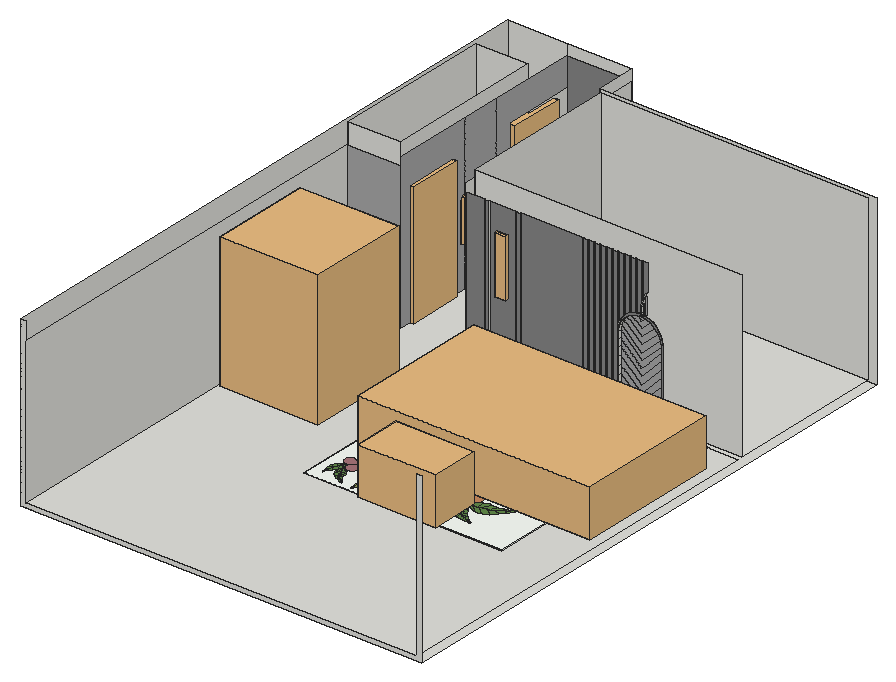
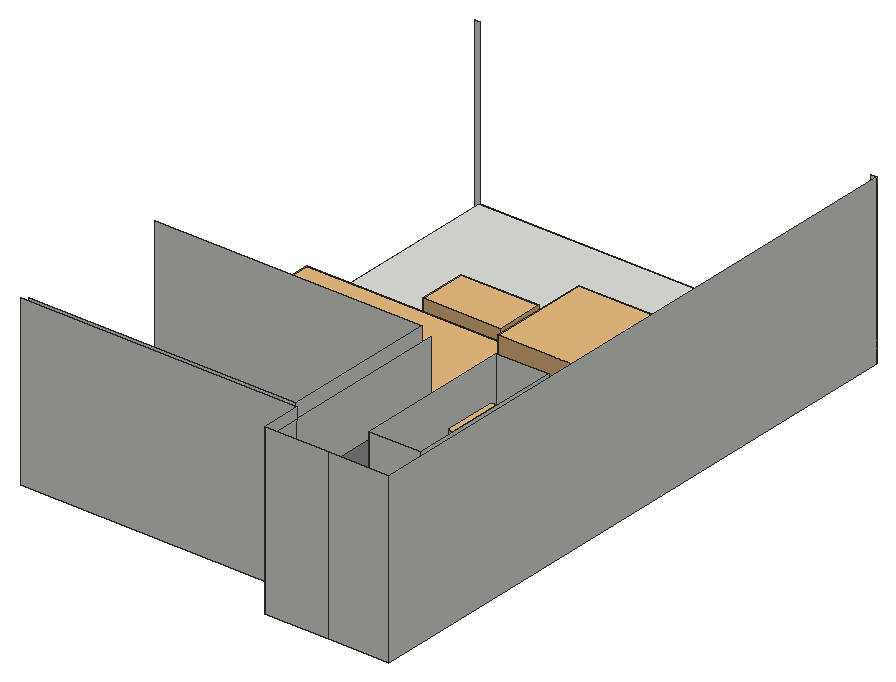
# SketchUp Ruby script. Lengths in inches.
U = 1.inch
M = Sketchup.active_model
def pt(a) = Geom::Point3d.new(a.map { |v| v * U })
def face(e, loops, mat)
  f = e.add_face(loops[0].map { |a| pt(a) })
  loops[1..].each { |l| e.add_face(l.map { |a| pt(a) }).erase! }
  f.material = f.back_material = mat if mat
  f
end
# faces: each face lists its corners as indices into pts; further lists are holes
def faces(e, pts, list, mat = nil) = list.each { |f| face(e, (f[0].is_a?(Array) ? f : [f]).map { |l| l.map { |i| pts[i] } }, mat) }
# xy, xz, yz: faces in a plane at the given z, y or x. An outline is a flat list of corners, or four numbers for a rectangle; further outlines are holes
def ring(l) = l.size == 4 ? [[l[0], l[1]], [l[2], l[1]], [l[2], l[3]], [l[0], l[3]]] : l.each_slice(2).to_a
def flat(e, list, mat, &to3) = list.each { |f| face(e, (f[0].is_a?(Array) ? f : [f]).map { |l| ring(l).map { |u, v| to3.(u, v) } }, mat) }
def xy(e, z, list, mat = nil) = flat(e, list, mat) { |x, y| [x, y, z] }
def xz(e, y, list, mat = nil) = flat(e, list, mat) { |x, z| [x, y, z] }
def yz(e, x, list, mat = nil) = flat(e, list, mat) { |y, z| [x, y, z] }
def lines(e, pts, list) = list.each { |a, b| e.add_line(pt(pts[a]), pt(pts[b])) }
# prism: a flat outline (further loops are holes) pulled along v
def prism(e, loops, v, mat = nil)
  f = face(e, loops, mat); d = Geom::Vector3d.new(v.map { |x| x * U })
  f.pushpull(f.normal.samedirection?(d) ? d.length : -d.length)
end
def box(e, o, s, mat = nil) = prism(e, [[o, [o[0] + s[0], o[1], o[2]], [o[0] + s[0], o[1] + s[1], o[2]], [o[0], o[1] + s[1], o[2]]]], [0, 0, s[2]], mat)
def at(x, y, z, deg = 0) = Geom::Transformation.translation(pt([x, y, z])) * Geom::Transformation.rotation(ORIGIN, Z_AXIS, deg.degrees)
def axes(o, x, y, z) = Geom::Transformation.new([*x, 0, *y, 0, *z, 0, *pt(o).to_a, 1])
def part(name) = M.definitions.add(name)
# library, detail: a bought-in or finely detailed component or shape, given as its bounding box
def library(name, o, s) = part(name).tap { |d| box(d.entities, o, s) }
def detail(e, o, s) = box(e.add_group.entities, o, s)
def put(e, d, t, mat = nil) = e.add_instance(d, t).tap { |i| i.material = mat if mat }
def group(e, t, mat = nil) = e.add_group.tap { |g| g.transformation = t; g.material = mat if mat }.entities
root = M.entities
M.materials.add("[0013_LightCoral]").color = [251, 255, 248]
M.materials.add("[0013_LightCoral]1").color = [240, 128, 128]
M.materials.add("[0132_LightGray]").color = [135, 135, 135]
M.materials.add("[0132_LightGray]1").color = [169, 169, 169]
M.materials.add("[Fabric Linen]").color = [168, 116, 117]
M.materials.add("[Granite Tile]").color = [201, 139, 95]
M.materials.add("[Vegetation Blur 01]").color = [168, 117, 122]
M.materials.add("[Vegetation Grass Artificial]").color = [98, 140, 74]
M.materials.add("[Vegetation Grass]").color = [144, 160, 91]
c1 = library("Dining+table+4+seater",[21.1,70.47,0],[72.14,73.92,98.58])
c2 = library("door (1)",[38.93,25.48,0],[40,9.94,82.68])
c3 = library("Succulent+decoration+(1)",[22.63,43.09,0],[32.53,2.35,30.92])
c4 = part("Group\#33")
xy(c4.entities,0,[[3.16,0,2.86,0.82,1.26,2.77,0,5.57,0.11,6.86,0.4375,6.76,0.52,6.68,0.63,6.49,1.02,6.09,1.86,5.44,2.36,5.07,2.77,4.84,3.39,4.72,3.7,4.65,4.07,4.27,3.85,2.85,3.75,2.45],[3.16,0,3.75,2.45,4.12,2.5,4.33,2.64,4.83,2.9,6,3.45,6.93,3.96,7.42,4.13,7.62,4.24,7.93,4.17,7.65,3.64,5.62,1.44],[3.75,2.45,3.85,2.85,4.07,4.27,4.28,5.69,4.62,5.72,4.99,5.91,5.7,6.28,6.96,7,8.1,7.62,9.16,8.86,9.08,6.35,8.01,4.32,7.93,4.17,7.62,4.24,7.42,4.13,6.93,3.96,6,3.45,4.83,2.9,4.33,2.64,4.12,2.5],[4.07,4.27,3.7,4.65,3.39,4.72,2.77,4.84,2.36,5.07,1.86,5.44,1.02,6.09,0.63,6.49,0.52,6.68,0.4375,6.76,0.11,6.86,0.14,7.22,0.28,8.87,0.86,10.33,1.05,9.89,1.35,9.64,1.86,9.3125,2.43,9.02,2.94,8.61,3.51,7.66,3.92,7.21,4.43,6.89,4.28,5.69],[4.28,5.69,4.43,6.89,4.58,8.08,4.59,8.84,4.91,8.96,5.15,9.24,5.74,9.79,6.26,10.125,6.8,10.3125,7.37,10.58,7.8,10.9,8.23,11.24,8.64,11.89,9.16,8.86,8.1,7.62,6.96,7,5.7,6.28,4.99,5.91,4.62,5.72],
  [4.43,6.89,3.92,7.21,3.51,7.66,2.94,8.61,2.43,9.02,1.86,9.3125,1.35,9.64,1.05,9.89,0.86,10.33,1.44,11.8,1.87,13.11,2.28,13.24,2.5,13.125,2.83,12.88,3.0625,12.74,3.16,12.51,3.3,12.2,3.96,11.625,4.28,11.32,4.5,11.15,4.6,11.16,4.61,10.45,4.59,8.84,4.58,8.08],[4.59,8.84,4.61,10.45,4.6,11.16,4.58,12.86,4.66,13.19,4.88,13.24,5.22,13.32,5.85,13.71,6.06,14.02,6.21,14.38,6.39,14.7,6.78,15.17,7.14,14.6,8.64,11.89,8.23,11.24,7.8,10.9,7.37,10.58,6.8,10.3125,6.26,10.125,5.74,9.79,5.15,9.24,4.91,8.96],[4.5,11.15,4.28,11.32,3.96,11.625,3.3,12.2,3.16,12.51,3.0625,12.74,2.83,12.88,2.5,13.125,2.28,13.24,1.87,13.11,2.29,14.41,2.4,16.15,3.04,16.01,3.53,15.76,4.54,15.27,4.58,12.86,4.6,11.16],[4.58,12.86,4.54,15.27,3.82,17.41,3.98,17.35,4.0625,17.43,4.29,17.71,4.85,18.28,6.78,15.17,6.39,14.7,6.21,14.38,6.06,14.02,5.85,13.71,5.22,13.32,4.88,13.24,4.66,13.19],[4.54,15.27,3.53,15.76,3.04,16.01,2.4,16.15,2.51,17.89,2.36,19.5,3.27,19.22,3.62,18.5625,3.82,17.41],
  [3.98,17.35,3.82,17.41,3.62,18.5625,3.27,19.22,2.97,19.94,2.74,20.53,2.73,21.38,3.15,20.92,4.15,19.41,4.85,18.28,4.29,17.71,4.0625,17.43],[3.27,19.22,2.36,19.5,2.21,21.11,2.74,20.53,2.97,19.94],[2.74,20.53,2.21,21.11,2.22,21.31,2.1875,21.5,2.16,21.66,2.15,21.73,2.13,21.81,2.18,21.79,2.45,21.6,2.6,21.53,2.73,21.38]])
c5 = part("Group\#60")
g1 = group(c5.entities,at(9.35,11.87,0))
xy(g1,0,[[2.08,-11.87,1.91,-11.81,1.82,-11.79,1.73,-11.73,1.59,-11.28,1.96,-11.51,1.99,-11.61,2.03,-11.71,2.1,-11.85,2.1,-11.87],[1.73,-11.73,1.4375,-11.55,0.68,-10.9,0.14,-10.4,0.36,-10.02,0.43,-9.83,0.47,-9.78,0.56,-9.79,0.84,-10.37,1.12,-10.67,1.38,-11,1.59,-11.28],[1.96,-11.51,1.59,-11.28,1.38,-11,1.12,-10.67,1.64,-10.68],[1.64,-10.68,1.12,-10.67,0.84,-10.37,0.56,-9.79,-0.14,-8.76,0.47,-8.87,0.76,-8.93,1.125,-8.91,1.32,-9.85],[0.14,-10.4,-1.34,-9.04,-1.2,-8.73,-1.16,-8.54,-1.13,-8.32,-1.0625,-8.13,-0.79,-7.83,-0.62,-7.74,-0.51,-7.68,-0.52,-7.49,-0.14,-8.76,0.56,-9.79,0.47,-9.78,0.43,-9.83,0.36,-10.02],
  [-1.34,-9.04,-1.62,-8.79,-2.81,-7.58,-2.69,-7.17,-2.52,-6.93,-2.33,-6.69,-2.07,-6.47,-1.81,-6.29,-1.59,-6.04,-1.36,-5.66,-1.27,-5.47,-1.12,-5.36,-0.89,-6.22,-0.78,-6.59,-0.52,-7.49,-0.51,-7.68,-0.62,-7.74,-0.79,-7.83,-1.0625,-8.13,-1.13,-8.32,-1.16,-8.54,-1.2,-8.73],[0.76,-8.93,0.47,-8.87,-0.14,-8.76,-0.52,-7.49,-0.78,-6.59,-0.73,-6.57,-0.59,-6.63,-0.37,-6.74,0.0625,-6.95,0.18,-7.09,0.27,-7.2,0.41,-7.24,0.62,-7.32,0.75,-7.35,0.96,-7.22,0.92,-7.97,1.125,-8.91],[-2.81,-7.58,-3.54,-6.05,-3.16,-5.24,-2.65,-4.74,-2.09,-4.17,-1.77,-3.87,-1.6,-3.71,-1.42,-3.65,-1.33,-4.31,-1.23,-4.96,-1.12,-5.36,-1.27,-5.47,-1.36,-5.66,-1.59,-6.04,-1.81,-6.29,-2.07,-6.47,-2.33,-6.69,-2.52,-6.93,-2.69,-7.17],[0.75,-7.35,0.62,-7.32,0.41,-7.24,0.27,-7.2,0.18,-7.09,0.0625,-6.95,-0.37,-6.74,-0.59,-6.63,-0.73,-6.57,-0.78,-6.59,-0.89,-6.22,-1.12,-5.36,-1.23,-4.96,-1.33,-4.31,-1.01,-4.4,-0.72,-4.58,-0.28,-5,0.05,-5.14,0.4,-5.21,0.71,-5.31,0.91,-5.4,1.08,-5.6,0.99,-6.46,0.96,-7.22],[-3.54,-6.05,-3.87,-4.71,-3.6,-3.47,-3.58,-3.39,-3.41,-3.375,-3.32,-3.29,-3.08,-3.13,-2.67,-2.72,-2.13,-2.25,-1.9,-2.04,-1.8125,-1.9375,-1.625,-1.85,-1.62,-2.08,-1.52,-2.86,-1.42,-3.65,-1.6,-3.71,-1.77,-3.87,-2.09,-4.17,-2.65,-4.74,-3.16,-5.24],
  [1.08,-5.6,0.91,-5.4,0.71,-5.31,0.4,-5.21,0.05,-5.14,-0.28,-5,-0.72,-4.58,-1.01,-4.4,-1.33,-4.31,-1.42,-3.65,-1.52,-2.86,-1.27,-3.01,-1.09,-3,-0.75,-2.98,-0.5,-3.04,-0.18,-3.16,0.36,-3.375,0.63,-3.53,0.72,-3.61,0.77,-3.64,0.96,-3.65,1,-3.84,1.17,-4.74],[0.96,-3.65,0.77,-3.64,0.72,-3.61,0.63,-3.53,0.36,-3.375,-0.18,-3.16,-0.5,-3.04,-0.75,-2.98,-1.09,-3,-1.27,-3.01,-1.52,-2.86,-1.62,-2.08,-1.625,-1.85,-1.67,-0.47,-1.39,-0.86,-0.26,-1.66,0.83,-2.95],[-3.58,-3.39,-3.51,-3.0625,-2.76,-1.6,-1.67,-0.47,-1.625,-1.85,-1.8125,-1.9375,-1.9,-2.04,-2.13,-2.25,-2.67,-2.72,-3.08,-3.13,-3.32,-3.29,-3.41,-3.375]])
put(c5.entities,c4,axes([8.26,10.79,0],[-0.18907,0.36013,0],[-0.36013,-0.18907,0],[0,0,1]))
c6 = library("Group\#329",[0,0,0],[7.875,1.97,42.125])
c7 = part("Group\#34")
xy(c7.entities,0,[[9.92,0,2.48,3.46,1.45,4.25,0.66,5.28,0.17,6.47,0,7.76,0.17,9.04,0.66,10.24,1.45,11.26,2.48,12.05,3.68,12.55,4.96,12.72,6.24,12.55,7.44,12.05,8.47,11.26,9.26,10.24,9.75,9.04,9.92,7.76]])
c8 = part("Group\#36")
xy(c8.entities,0,[[9.92,0,2.48,3.46,1.45,4.25,0.66,5.28,0.17,6.47,0,7.76,0.17,9.04,0.66,10.24,1.45,11.26,2.48,12.05,3.68,12.55,4.96,12.72,6.24,12.55,7.44,12.05,8.47,11.26,9.26,10.24,9.75,9.04,9.92,7.76]])
c9 = part("Group\#38")
put(c9.entities,c4,at(-0.96,4.16,0,-54.9))
put(c9.entities,c4,at(0.46,7.11,0,4.699))
c10 = library("Throw pillow",[0,0,0],[9.42,19.46,15.55])
c11 = library("Group\#76",[0,0,0],[62.16,38.23,37.78])
c12 = library("sofa",[-89.99,-57.625,20.49],[181.58,106.54,46.48])
box(root,[107.14,126.82,3.125],[145.28,96.85,0.4375],"[0013_LightCoral]")
xy(root,0,[[0,0,44.125,447.875],[44.125,0,91.5625,447.875],[91.5625,0,295.1875,417.6875]])
xy(root,3.125,[[3.79,0,291.63,0,291.63,294.91,278.7,294.91,278.7,294.47,277.02,294.47,277.02,294.91,276.67,294.91,276.67,294.47,274.98,294.47,274.98,294.91,274.63,294.91,274.63,294.47,272.94,294.47,272.94,294.91,272.59,294.91,272.59,294.47,270.9,294.47,270.9,294.91,270.55,294.91,270.55,294.47,268.86,294.47,268.86,294.91,268.52,294.91,268.52,294.47,266.83,294.47,266.83,294.91,266.48,294.91,266.48,294.47,264.79,294.47,264.79,294.91,264.44,294.91,264.44,294.47,260.79,294.47,260.79,294.91,260.26,294.91,260.26,294.47,257.75,294.47,257.75,293.53,204.25,293.53,204.25,294.91,203.53,294.91,203.53,294.47,199.88,294.47,199.88,294.91,199.15,294.91,199.15,294.47,195.5,294.47,195.5,294.91,194.78,294.91,194.78,294.47,191.13,294.47,191.13,294.91,190.4,294.91,190.4,294.47,186.75,294.47,186.75,294.91,186.03,294.91,186.03,294.47,182.38,294.47,182.38,294.91,181.65,294.91,181.65,294.47,178,294.47,178,294.91,132.13,294.91,132.13,294.47,129.06,294.47,129.06,294.91,109.17,294.91,109.17,294.47,105.89,294.47,105.89,294.91,91.5625,294.91,91.5625,447.375,44.125,447.375,44.125,294.91,3.79,294.91],[2.9,297.81,41.22,414.79],[95.12,298.46,291.63,414.13],[41.22,302.6,44.125,342.1],[41.22,394.68,44.125,412.06]])
xy(root,4.38,[[205.51,293.53,236.48,294.91]],"[0132_LightGray]")
xy(root,74.29,[[216.65,293.53,216.66,294.91]])
xy(root,74.86,[[220.99,293.53,221.03,294.91]])
xz(root,0,[[0,0,295.1875,0,295.1875,123.125,291.63,123.125,291.63,3.125,3.79,3.125,3.79,123.125,0,123.125]])
xz(root,293.53,[[[204.25,3.125,237.73,3.125,237.73,58.125,237.16,62.46,236.33,64.45,235.49,66.49,233.34,69.3,232.83,69.96,230.15,72.02,229.36,72.62,227.05,73.58,225.4,74.26,225.32,74.29,225.04,74.33,222.99,74.6,222.32,74.6875,221.75,74.76,221.03,74.86,220.99,74.86,217.38,74.39,216.66,74.29,216.65,74.29,213,72.78,212.625,72.62,212.28,72.36,209.16,69.96,208.63,69.27,207.9,68.33,206.5,66.49,204.82,62.46,204.25,58.125],[205.51,4.38,205.51,58.04,206.04,62.13,207.59,65.86,208.9,67.5625,209.625,68.51,210.05,69.07,213.04,71.36,213.25,71.53,213.48,71.62,216.99,73.07,217.54,73.15,220.99,73.6,221.59,73.52,225,73.07,228.73,71.53,231.93,69.07,234.39,65.86,235.94,62.13,236.48,58.04,236.48,4.38]]],"[0132_LightGray]")
xz(root,294.47,[[105.89,3.125,109.17,109.39],[129.06,3.125,132.13,109.39],[178,3.125,181.65,109.39],[182.38,3.125,186.03,109.39],[186.75,3.125,190.4,109.39],
  [191.13,3.125,194.78,109.39],[195.5,3.125,199.15,109.39],[199.88,3.125,203.53,109.39],[204.25,58.125,204.82,62.46,206.5,66.49,207.9,68.33,207.9,109.39,204.25,109.39],[208.63,69.27,209.16,69.96,212.28,72.36,212.28,109.39,208.63,109.39],
  [213,72.78,216.65,74.29,216.65,109.39,213,109.39],[217.38,74.39,220.99,74.86,220.99,80.18,221.03,80.29,221.03,109.39,217.38,109.39],[221.75,82.74,222.51,85.27,225.4,89.72,225.4,109.39,221.75,109.39]],"[0132_LightGray]")
xz(root,294.66,[[225.04,74.33,225.04,86.79,223.69,84.72,223.11,82.79,223.11,74.58],[222.99,74.6,222.99,82.375,222.32,80.11,222.32,74.6875]],"[0132_LightGray]1")
xz(root,294.91,[[223.11,74.58,223.11,82.79,222.99,82.375,222.99,74.6],[220.99,74.86,221.03,74.86,221.03,80.29,220.99,80.18]])
xz(root,294.91,[[91.5625,3.125,105.89,109.39],[109.17,3.125,129.06,109.39],[132.13,3.125,178,109.39],[181.65,3.125,182.38,109.39],[186.03,3.125,186.75,109.39],
  [190.4,3.125,191.13,109.39],[194.78,3.125,195.5,109.39],[199.15,3.125,199.88,109.39],[203.53,3.125,204.25,109.39],[205.51,4.38,220.99,4.38,205.51,17.84],
  [220.99,4.38,236.48,17.84,236.48,25.84,220.99,10.29,205.51,23.88,205.51,17.84],[207.9,68.33,208.63,69.27,208.63,109.39,207.9,109.39],[212.28,72.36,212.625,72.62,213,72.78,213,109.39,212.28,109.39],[216.65,74.29,216.66,74.29,217.38,74.39,217.38,109.39,216.65,109.39],[221.03,80.29,221.75,82.74,221.75,109.39,221.03,109.39]],"[0132_LightGray]")
xz(root,294.91,[[3.79,3.125,44.125,109.39],[220.99,10.29,236.48,25.84,236.48,31.64,220.99,16.21,205.51,29.28,205.51,23.88],[220.99,16.21,236.48,31.64,236.48,37.31,220.99,21.66,205.51,35.56,205.51,29.28],[220.99,21.66,236.48,37.31,236.48,43.35,220.99,27.22,205.51,42.09,205.51,35.56],[220.99,27.22,236.48,43.35,236.48,48.5,220.99,32.74,205.51,47.96,205.51,42.09],
  [220.99,32.74,236.48,48.5,236.48,54.0625,220.99,38.12,205.51,53.16,205.51,47.96],[220.99,38.12,236.48,54.0625,236.48,58.04,220.99,43.39,205.51,58.04,205.51,53.16],[220.99,43.39,236.48,58.04,235.94,62.13,220.99,48.55,206.04,62.13,205.51,58.04],[220.99,48.55,235.94,62.13,234.39,65.86,220.99,53.67,207.59,65.86,206.04,62.13],[220.99,53.67,234.39,65.86,231.93,69.07,220.99,58.89,210.05,69.07,209.625,68.51,208.9,67.5625,207.59,65.86],
  [220.99,58.89,231.93,69.07,228.73,71.53,220.99,64.73,213.25,71.53,213.04,71.36,210.05,69.07],[220.99,64.73,228.73,71.53,225,73.07,220.99,69.26,216.99,73.07,213.48,71.62,213.25,71.53],[220.99,69.26,225,73.07,221.59,73.52,220.99,73.6,217.54,73.15,216.99,73.07]],"[0132_LightGray]1")
xz(root,297.81,[[2.9,3.125,41.22,123.125]])
xz(root,298.46,[[95.12,3.125,291.63,123.125]])
xz(root,302.6,[[41.22,3.125,44.125,93.25]])
xz(root,342.1,[[41.22,3.125,44.125,93.25]])
xz(root,394.68,[[41.22,3.125,44.125,93.9375]])
xz(root,412.06,[[41.22,3.125,44.125,93.9375]])
xz(root,414.13,[[95.12,3.125,291.63,123.125]])
xz(root,414.79,[[2.9,3.125,41.22,123.125]])
xz(root,417.6875,[[91.5625,0,295.1875,123.125]])
xz(root,447.375,[[44.125,3.125,91.5625,115.375]],"[0132_LightGray]")
xz(root,447.875,[[0,0,44.125,123.125],[44.125,0,91.5625,123.125]])
yz(root,0,[[0,0,447.875,123.125]])
yz(root,2.9,[[297.81,3.125,414.79,123.125]])
yz(root,3.79,[[0,3.125,294.91,109.39]])
yz(root,41.22,[[297.81,3.125,297.81,123.125,414.79,123.125,414.79,3.125,412.06,3.125,412.06,93.9375,394.68,93.9375,394.68,3.125,342.1,3.125,342.1,93.25,302.6,93.25,302.6,3.125]])
yz(root,44.125,[[381.77,3.125,381.96,115.375],[412.06,3.125,447.375,93.9375]])
yz(root,44.125,[[294.91,3.125,302.6,3.125,302.6,93.25,342.1,93.25,342.1,3.125,353.48,3.125,353.48,115.375,294.91,115.375],[353.48,3.125,381.77,115.375],[381.96,3.125,394.68,3.125,394.68,93.9375,447.375,93.9375,447.375,115.375,381.96,115.375]],"[0132_LightGray]1")
yz(root,91.5625,[[417.6875,0,447.875,0,447.875,123.125,417.6875,123.125,417.6875,115.375,447.375,115.375,447.375,3.125,417.6875,3.125],[294.91,3.125,417.6875,115.375],[417.6875,3.125,447.375,115.375]])
yz(root,95.12,[[298.46,3.125,414.13,123.125]])
yz(root,105.89,[[294.47,3.125,294.91,109.39]])
yz(root,109.17,[[294.47,3.125,294.91,109.39]])
yz(root,129.06,[[294.47,3.125,294.91,109.39]])
yz(root,132.13,[[294.47,3.125,294.91,109.39]])
yz(root,178,[[294.47,3.125,294.91,109.39]])
yz(root,181.65,[[294.47,3.125,294.91,109.39]])
yz(root,182.38,[[294.47,3.125,294.91,109.39]])
yz(root,186.03,[[294.47,3.125,294.91,109.39]])
yz(root,186.75,[[294.47,3.125,294.91,109.39]])
yz(root,190.4,[[294.47,3.125,294.91,109.39]])
yz(root,191.13,[[294.47,3.125,294.91,109.39]])
yz(root,194.78,[[294.47,3.125,294.91,109.39]])
yz(root,195.5,[[294.47,3.125,294.91,109.39]])
yz(root,199.15,[[294.47,3.125,294.91,109.39]])
yz(root,199.88,[[294.47,3.125,294.91,109.39]])
yz(root,203.53,[[294.47,3.125,294.91,109.39]])
yz(root,204.25,[[294.47,58.125,294.91,109.39]])
yz(root,204.25,[[293.53,3.125,294.91,58.125]],"[0132_LightGray]")
yz(root,205.51,[[293.53,4.38,294.91,17.84],[293.53,17.84,294.91,23.88],[293.53,23.88,294.91,29.28],[293.53,29.28,294.91,35.56],[293.53,35.56,294.91,42.09],
  [293.53,42.09,294.91,47.96],[293.53,47.96,294.91,53.16],[293.53,53.16,294.91,58.04]])
yz(root,207.9,[[294.47,68.33,294.91,109.39]])
yz(root,208.63,[[294.47,69.27,294.91,109.39]])
yz(root,212.28,[[294.47,72.36,294.91,109.39]])
yz(root,213,[[294.47,72.78,294.91,109.39]])
yz(root,216.65,[[294.47,74.29,294.91,109.39]])
yz(root,217.38,[[294.47,74.39,294.91,109.39]])
yz(root,220.99,[[294.47,74.86,294.91,80.18]])
yz(root,221.03,[[293.53,74.86,294.91,80.29],[294.47,80.29,294.91,109.39]])
yz(root,221.75,[[294.47,82.74,294.91,109.39]])
yz(root,222.32,[[293.53,74.6875,294.66,75.99],[293.53,75.99,294.66,80.11]])
yz(root,222.99,[[294.66,74.6,294.91,82.375]])
yz(root,223.11,[[294.66,74.58,294.91,82.79]])
p = [[205.51,294.91,58.04],[206.04,294.91,62.13],[206.04,293.53,62.13],[205.51,293.53,58.04],[204.82,293.53,62.46],[204.82,294.47,62.46],
  [204.25,294.47,58.125],[204.25,293.53,58.125],[207.59,294.91,65.86],[207.59,293.53,65.86],[206.5,293.53,66.49],[206.5,294.47,66.49],
  [208.9,294.91,67.5625],[208.9,293.53,67.5625],[207.9,293.53,68.33],[207.9,294.47,68.33],[209.625,294.91,68.51],[209.625,293.53,68.51],
  [208.63,294.91,69.27],[207.9,294.91,68.33],[208.63,293.53,69.27],[208.63,294.47,69.27],[210.05,294.91,69.07],[210.05,293.53,69.07],
  [213.04,294.91,71.36],[213.04,293.53,71.36],[209.16,293.53,69.96],[209.16,294.47,69.96],[212.28,293.53,72.36],[212.28,294.47,72.36],
  [213.25,294.91,71.53],[213.25,293.53,71.53],[213.48,294.91,71.62],[213.48,293.53,71.62],[216.99,294.91,73.07],[216.99,293.53,73.07],
  [212.625,294.91,72.62],[212.28,294.91,72.36],[212.625,293.53,72.62],[213,294.91,72.78],[213,293.53,72.78],[213,294.47,72.78],
  [216.65,293.53,74.29],[216.65,294.47,74.29],[217.54,294.91,73.15],[217.54,293.53,73.15],[220.99,294.91,73.6],[220.99,293.53,73.6],
  [221.59,294.91,73.52],[225,294.91,73.07],[225,293.53,73.07],[221.59,293.53,73.52],[217.38,294.91,74.39],[216.66,294.91,74.29],
  [216.66,293.53,74.29],[217.38,293.53,74.39],[217.38,294.47,74.39],[225.04,293.53,74.33],[225.04,294.66,74.33],[223.11,294.66,74.58],
  [223.11,294.91,74.58],[222.99,294.91,74.6],[222.99,294.66,74.6],[222.99,293.53,74.6],[220.99,293.53,74.86],[220.99,294.47,74.86],
  [222.32,294.66,74.6875],[222.32,293.53,74.6875],[222.32,293.53,80.11],[222.32,294.66,80.11],[222.99,294.66,82.375],[222.99,293.53,82.375],
  [220.99,294.91,80.18],[221.03,294.91,80.29],[221.03,294.47,80.29],[220.99,294.47,80.18],[221.75,294.91,82.74],[221.03,293.53,80.29],
  [221.75,293.53,82.74],[221.75,294.47,82.74],[222.99,294.91,82.375],[223.11,294.91,82.79],[223.11,294.66,82.79],[223.69,294.66,84.72],
  [223.69,293.53,84.72],[222.51,293.53,85.27],[222.51,294.47,85.27],[225.4,293.53,89.72],[225.4,294.47,89.72],[44.3125,353.48,115.375],
  [44.3125,353.48,3.125]]
faces(root,p,[[0,1,2,3],[4,5,6,7],[1,8,9,2],[10,11,5,4],[8,12,13,9],[14,15,11,10],[12,16,17,13],[18,19,15,14,20,21],
  [16,22,23,17],[22,24,25,23],[26,27,21,20],[28,29,27,26],[24,30,31,25],[30,32,33,31],[32,34,35,33],[36,37,29,28,38],
  [39,36,38,40,41],[42,43,41,40],[34,44,45,35],[44,46,47,45],[48,49,50,51],[46,48,51,47],[52,53,54,55,56],[57,58,59,60,61,62,63],
  [64,65,56,55],[63,62,66,67],[68,69,70,71],[72,73,74,75],[76,73,74,77,78,79],[80,81,82,83,84,71,70],[85,86,79,78],[87,88,86,85]])
lines(root,p,[[89,90]])
put(root,c1,at(-15.3,105.67,3.125))
put(root,c2,axes([72.34,263.67,3.125],[0,1,0],[-1,0,0],[0,0,1.09008]))
put(root,c2,axes([73.41,355.75,3.125],[0,1,0],[-1,0,0],[0,0,1.09008]))
put(root,c3,axes([89.57,319.11,34.0625],[0,1.37,0],[-1,0,0],[0,0,1]))
put(root,c5,axes([111.03,185.11,3.61],[0,-1.23,0],[1.23,0,0],[0,0,1.23]),"[Vegetation Grass]")
put(root,c6,at(115.17,292.28,49.76))
g2 = group(root,at(130.7,169.56,3.61),"[Vegetation Grass Artificial]")
put(g2,c4,axes([-6.94,-23.77,0],[-0.6328,-0.40312,0],[0.40312,-0.6328,0],[0,0,1.23]))
put(g2,c7,axes([2.27,-10.78,0],[-0.6637,-0.34993,0],[0.34993,-0.6637,0],[0,0,1.23]),"[Vegetation Blur 01]")
put(g2,c4,axes([-7.04,-21.32,0],[-0.66793,0.3418,0],[-0.3418,-0.66793,0],[0,0,1.23]))
put(g2,c8,axes([1.16,-19.29,0],[-0.55229,0.50786,0],[-0.50786,-0.55229,0],[0,0,1.23]),"[Vegetation Blur 01]")
put(g2,c8,axes([-5.22,-6.86,0],[0.09144,-0.74471,0],[0.74471,0.09144,0],[0,0,1.23]),"[Vegetation Blur 01]")
put(g2,c8,axes([-7.01,-21.19,0],[0.27133,0.69952,0],[-0.69952,0.27133,0],[0,0,1.23]),"[Vegetation Blur 01]")
put(g2,c8,axes([-11.68,-13.16,0],[0.74225,-0.10961,0],[0.10961,0.74225,0],[0,0,1.23]),"[Vegetation Blur 01]")
g3 = group(root,at(172.11,193.08,3.61),"[Vegetation Grass Artificial]")
put(g3,c9,axes([-30.02,12.46,0],[-0.71076,1.00385,0],[-1.00385,-0.71076,0],[0,0,1.23]))
g4 = group(g3,at(-22.77,22.5,0),"[Granite Tile]")
xy(g4,0,[[-4.25,-15.75,-8.57,-11.62,-9.45,-10.3,-9.96,-8.79,-10.0625,-7.2,-9.75,-5.64,-9.04,-4.21,-7.99,-3.01,-6.67,-2.13,-5.16,-1.62,-3.57,-1.51,-2.01,-1.83,-0.58,-2.53,0.62,-3.58,1.5,-4.91,2.01,-6.42,2.11,-8.01,1.8,-9.57,-0.07,-15.08,0.1,-14.2,0.06,-13.55,-0.15,-12.93,-0.51,-12.39,-1.01,-11.95,-1.59,-11.66,-2.24,-11.54,-2.89,-11.58,-3.51,-11.79,-4.05,-12.15,-4.49,-12.64,-4.78,-13.23,-4.9,-13.87,-4.86,-14.53,-4.65,-15.15]])
xy(g4,0,[[-1.27,-18.6,-4.25,-15.75,-4.65,-15.15,-4.86,-14.53,-4.9,-13.87,-4.78,-13.23,-4.49,-12.64,-4.05,-12.15,-3.51,-11.79,-2.89,-11.58,-2.24,-11.54,-1.59,-11.66,-1.01,-11.95,-0.51,-12.39,-0.15,-12.93,0.06,-13.55,0.1,-14.2,-0.07,-15.08]],"[Fabric Linen]")
g5 = group(g3,at(-41.24,11.1,0),"[Granite Tile]")
xy(g5,0,[[5.11,-12.26,3.57,-11.85,2.19,-11.05,1.07,-9.92,0.27,-8.54,-0.13,-7,-0.13,-5.41,0.28,-3.87,1.08,-2.49,2.21,-1.37,3.59,-0.57,5.13,-0.16,6.72,-0.16,8.26,-0.58,9.64,-1.38,14.25,-4.93,13.48,-4.48,12.85,-4.3125,12.19,-4.31,11.56,-4.48,10.99,-4.81,10.53,-5.27,10.2,-5.83,10.03,-6.47,10.03,-7.12,10.2,-7.75,10.52,-8.32,10.98,-8.78,11.55,-9.11,12.18,-9.28,12.84,-9.28,13.55,-9.1,8.24,-11.85,6.7,-12.26]])
xy(g5,0,[[12.18,-9.28,11.55,-9.11,10.98,-8.78,10.52,-8.32,10.2,-7.75,10.03,-7.12,10.03,-6.47,10.2,-5.83,10.53,-5.27,10.99,-4.81,11.56,-4.48,12.19,-4.31,12.85,-4.3125,13.48,-4.48,14.25,-4.93,17.2,-7.2,13.55,-9.1,12.84,-9.28]],"[Fabric Linen]")
g6 = group(g3,at(-14.25,-11.97,0),"[Granite Tile]")
xy(g6,0,[[-1,2.4,-2.59,2.55,-4.08,3.12,-5.37,4.05,-6.38,5.28,-7.04,6.73,-8.72,12.3,-8.35,11.49,-7.9375,10.98,-7.4,10.6,-6.79,10.37,-6.14,10.31,-5.49,10.41,-4.9,10.68,-4.39,11.1,-4.01,11.63,-3.78,12.24,-3.71,12.89,-3.82,13.54,-4.09,14.13,-4.5,14.64,-5.03,15.02,-5.72,15.28,0.2,14.44,1.6875,13.87,2.98,12.94,3.99,11.71,4.65,10.26,4.9,8.6875,4.75,7.1,4.18,5.61,3.25,4.32,2.02,3.31,0.57,2.65]])
xy(g6,0,[[-6.14,10.31,-6.79,10.37,-7.4,10.6,-7.9375,10.98,-8.35,11.49,-8.72,12.3,-9.79,15.86,-5.72,15.28,-5.03,15.02,-4.5,14.64,-4.09,14.13,-3.82,13.54,-3.71,12.89,-3.78,12.24,-4.01,11.63,-4.39,11.1,-4.9,10.68,-5.49,10.41]],"[Fabric Linen]")
g7 = group(g3,at(-36.4,-10.0625,0),"[Granite Tile]")
xy(g7,0,[[8.17,-2.49,6.58,-2.38,5.07,-1.87,3.75,-0.98,2.71,0.22,2,1.65,1.7,3.22,1.81,4.8,2.32,6.3125,3.21,7.63,4.41,8.68,9.26,11.9,8.59,11.32,8.22,10.77,8.01,10.15,7.96,9.5,8.09,8.86,8.38,8.27,8.81,7.78,9.35,7.41,9.97,7.2,10.625,7.15,11.27,7.28,11.86,7.57,12.35,8,12.71,8.54,12.93,9.16,12.98,9.89,13.875,3.98,13.77,2.39,13.25,0.89,12.36,-0.4375,11.16,-1.48,9.73,-2.18]])
xy(g7,0,[[10.625,7.15,9.97,7.2,9.35,7.41,8.81,7.78,8.38,8.27,8.09,8.86,7.96,9.5,8.01,10.15,8.22,10.77,8.59,11.32,9.26,11.9,12.36,13.96,12.98,9.89,12.93,9.16,12.71,8.54,12.35,8,11.86,7.57,11.27,7.28]],"[Fabric Linen]")
g8 = group(g3,at(-5.95,8.4,0),"[Granite Tile]")
xy(g8,0,[[-8.55,-4.66,-14.37,-4.5625,-13.49,-4.46,-12.875,-4.22,-12.35,-3.83,-11.94,-3.32,-11.68,-2.72,-11.59,-2.07,-11.66,-1.42,-11.91,-0.81,-12.3,-0.28,-12.81,0.12,-13.41,0.38,-14.06,0.48,-14.71,0.4,-15.32,0.16,-15.84,-0.23,-16.3,-0.8,-13.69,4.58,-12.7,5.83,-11.42,6.78,-9.94,7.36,-8.36,7.55,-6.78,7.3125,-5.32,6.68,-4.07,5.69,-3.125,4.41,-2.54,2.93,-2.35,1.35,-2.59,-0.23,-3.22,-1.6875,-4.21,-2.9375,-5.49,-3.89,-6.97,-4.47]])
xy(g8,0,[[-14.37,-4.5625,-18.09,-4.51,-16.3,-0.8,-15.84,-0.23,-15.32,0.16,-14.71,0.4,-14.06,0.48,-13.41,0.38,-12.81,0.12,-12.3,-0.28,-11.91,-0.81,-11.66,-1.42,-11.59,-2.07,-11.68,-2.72,-11.94,-3.32,-12.35,-3.83,-12.875,-4.22,-13.49,-4.46]],"[Fabric Linen]")
put(root,c5,axes([129.52,139.42,3.61],[0.86974,-0.86974,0],[0.86974,0.86974,0],[0,0,1.23]),"[Vegetation Grass]")
put(root,c10,at(141.56,252.06,18.96,-93.3))
g9 = group(root,at(170.48,126.99,3.61),"[Vegetation Grass Artificial]")
put(g9,c4,axes([-11.87,30.73,0],[0.34295,0.93712,0],[-0.93712,0.34295,0],[0,0,1.23]))
put(g9,c7,axes([-11.11,9.56,0],[0.41857,0.90587,0],[-0.90587,0.41857,0],[0,0,1.23]),"[Vegetation Blur 01]")
put(g9,c4,axes([-9.79,28.21,0],[0.98182,0.17843,0],[-0.17843,0.98182,0],[0,0,1.23]))
put(g9,c8,axes([-16.8125,19.44,0],[0.99379,-0.09044,0],[0.09044,0.99379,0],[0,0,1.23]),"[Vegetation Blur 01]")
put(g9,c8,axes([-0.03,11.47,0],[-0.69819,0.71297,0],[-0.71297,-0.69819,0],[0,0,1.23]),"[Vegetation Blur 01]")
put(g9,c8,axes([-9.72,28.05,0],[0.2784,-0.95828,0],[0.95828,0.2784,0],[0,0,1.23]),"[Vegetation Blur 01]")
put(g9,c8,axes([1.71,23.34,0],[-0.87278,-0.48379,0],[0.48379,-0.87278,0],[0,0,1.23]),"[Vegetation Blur 01]")
put(root,c5,axes([173.11,206.33,3.61],[0.40856,1.16016,0],[-1.16016,0.40856,0],[0,0,1.23]),"[Vegetation Grass]")
put(root,c11,axes([150.63,122.02,4.84],[0.918,0,0],[0,0.918,0],[0,0,0.918]))
g10 = group(root,at(194.08,214.94,3.61),"[Vegetation Grass Artificial]")
put(g10,c4,axes([-15.8125,-13.23,0],[-0.62446,0.01418,0],[-0.01418,-0.62446,0],[0,0,1.23]))
put(g10,c7,axes([-3.42,-8.51,0],[-0.6212,0.06529,0],[-0.06529,-0.6212,0],[0,0,1.23]),"[Vegetation Blur 01]")
put(g10,c4,axes([-14.74,-11.49,0],[-0.30378,0.54578,0],[-0.54578,-0.30378,0],[0,0,1.23]))
put(g10,c8,axes([-8.13,-13.88,0],[-0.14688,0.60711,0],[-0.60711,-0.14688,0],[0,0,1.23]),"[Vegetation Blur 01]")
put(g10,c8,axes([-6.79,-2.33,0],[-0.28163,-0.55753,0],[0.55753,-0.28163,0],[0,0,1.23]),"[Vegetation Blur 01]")
put(g10,c8,axes([-14.66,-11.42,0],[0.51166,0.35827,0],[-0.35827,0.51166,0],[0,0,1.23]),"[Vegetation Blur 01]")
put(g10,c8,axes([-14.18,-3.7,0],[0.46272,-0.41957,0],[0.41957,0.46272,0],[0,0,1.23]),"[Vegetation Blur 01]")
put(root,c5,axes([178.9375,144.89,3.61],[0,-1.23,0],[1.23,0,0],[0,0,1.23]),"[Vegetation Grass]")
put(root,c12,axes([199.7,225.68,-11.7],[-0.94,0,0],[0,1,0],[0,0,0.75]),"[0013_LightCoral]1")
g11 = group(root,at(167.01,182.92,3.61),"[Vegetation Grass Artificial]")
put(g11,c9,axes([25.98,-24.09,0],[0.347,-1.29502,0],[1.29502,0.347,0],[0,0,1.23]))
g12 = group(g11,at(14.77,-31.61,0),"[Granite Tile]")
xy(g12,0,[[7.62,-0.35,5.89,-0.3,4.22,0.2,2.74,1.11,1.55,2.37,0.72,3.9,0.32,5.59,0.37,7.32,0.87,8.98,1.78,10.46,5.78,15.39,5.27,14.56,5.06,13.875,5.04,13.16,5.21,12.47,5.55,11.84,6.04,11.32,6.65,10.95,7.33,10.74,8.04,10.72,8.74,10.89,9.37,11.23,9.89,11.72,10.26,12.33,10.46,13.01,10.48,13.72,10.3,14.5,13.15,8.64,13.55,6.95,13.5,5.22,13.01,3.55,12.1,2.07,10.84,0.88,9.31,0.06]])
xy(g12,0,[[8.04,10.72,7.33,10.74,6.65,10.95,6.04,11.32,5.55,11.84,5.21,12.47,5.04,13.16,5.06,13.875,5.27,14.56,5.78,15.39,8.33,18.53,10.3,14.5,10.48,13.72,10.46,13.01,10.26,12.33,9.89,11.72,9.37,11.23,8.74,10.89]],"[Fabric Linen]")
g13 = group(g11,at(37.96,-26.9375,0),"[Granite Tile]")
xy(g13,0,[[-3.45,1.94,-5.18,2.11,-6.8125,2.71,-8.23,3.72,-9.33,5.05,-12.7,10.43,-12.08,9.68,-11.5,9.27,-10.83,9.02,-10.125,8.95,-9.42,9.07,-8.77,9.37,-8.22,9.82,-7.81,10.4,-7.56,11.07,-7.49,11.78,-7.61,12.49,-7.91,13.13,-8.36,13.68,-8.94,14.1,-9.61,14.35,-10.41,14.42,-3.94,15.23,-2.21,15.07,-0.59,14.47,0.83,13.46,1.94,12.12,2.66,10.54,2.95,8.83,2.78,7.1,2.18,5.48,1.17,4.0625,-0.16,2.95,-1.74,2.23]])
xy(g13,0,[[-10.125,8.95,-10.83,9.02,-11.5,9.27,-12.08,9.68,-12.7,10.43,-14.86,13.86,-10.41,14.42,-9.61,14.35,-8.94,14.1,-8.36,13.68,-7.91,13.13,-7.61,12.49,-7.49,11.78,-7.56,11.07,-7.81,10.4,-8.22,9.82,-8.77,9.37,-9.42,9.07]],"[Fabric Linen]")
g14 = group(g11,at(19.09,6.85,0),"[Granite Tile]")
xy(g14,0,[[0.07,-17.78,-5.66,-14.68,-6.97,-13.54,-7.94,-12.1,-8.51,-10.46,-8.63,-8.73,-8.3,-7.03,-7.54,-5.47,-6.4,-4.15,-4.96,-3.18,-3.32,-2.62,-1.59,-2.5,0.12,-2.83,1.68,-3.59,2.99,-4.73,3.96,-6.17,4.53,-7.81,4.65,-9.54,4.26,-15.87,4.19,-14.9,3.96,-14.23,3.56,-13.64,3.02,-13.17,2.38,-12.86,1.68,-12.72,0.97,-12.77,0.29,-13,-0.3,-13.4,-0.77,-13.94,-1.08,-14.58,-1.22,-15.28,-1.17,-15.99,-0.93,-16.67,-0.54,-17.26]])
xy(g14,0,[[4.01,-19.92,0.07,-17.78,-0.54,-17.26,-0.93,-16.67,-1.17,-15.99,-1.22,-15.28,-1.08,-14.58,-0.77,-13.94,-0.3,-13.4,0.29,-13,0.97,-12.77,1.68,-12.72,2.38,-12.86,3.02,-13.17,3.56,-13.64,3.96,-14.23,4.19,-14.9,4.26,-15.87]],"[Fabric Linen]")
g15 = group(g11,at(41.01,-3.48,0),"[Granite Tile]")
xy(g15,0,[[-13.96,-8.67,-13.06,-8.32,-12.48,-7.9,-12.03,-7.35,-11.73,-6.7,-11.62,-5.99,-11.69,-5.28,-11.95,-4.62,-12.36,-4.04,-12.92,-3.59,-13.57,-3.29,-14.27,-3.18,-14.98,-3.25,-15.65,-3.51,-16.23,-3.92,-16.68,-4.48,-17.01,-5.2,-15.69,1.18,-14.98,2.76,-13.88,4.11,-12.47,5.12,-10.85,5.74,-9.125,5.91,-7.41,5.64,-5.83,4.92,-4.48,3.83,-3.47,2.42,-2.85,0.8,-2.67,-0.93,-2.95,-2.64,-3.66,-4.23,-4.76,-5.57,-6.17,-6.59,-7.79,-7.21]])
xy(g15,0,[[-17.91,-9.6,-17.01,-5.2,-16.68,-4.48,-16.23,-3.92,-15.65,-3.51,-14.98,-3.25,-14.27,-3.18,-13.57,-3.29,-12.92,-3.59,-12.36,-4.04,-11.95,-4.62,-11.69,-5.28,-11.62,-5.99,-11.73,-6.7,-12.03,-7.35,-12.48,-7.9,-13.06,-8.32,-13.96,-8.67]],"[Fabric Linen]")
g16 = group(g11,at(2.9,-10.84,0),"[Granite Tile]")
xy(g16,0,[[7.38,-11.29,5.69,-10.875,4.17,-10.04,2.91,-8.84,2.01,-7.36,1.53,-5.69,1.49,-3.96,1.9,-2.27,2.73,-0.75,3.93,0.51,5.41,1.41,7.08,1.9,8.82,1.9375,10.5,1.53,16.42,-0.77,15.47,-0.54,14.76,-0.55,14.08,-0.76,13.47,-1.125,12.97,-1.64,12.63,-2.27,12.46,-2.96,12.48,-3.67,12.68,-4.36,13.05,-4.97,13.5625,-5.46,14.19,-5.81,14.88,-5.97,15.6,-5.96,16.28,-5.76,16.96,-5.34,12.27,-9.86,10.78,-10.76,9.12,-11.25]])
xy(g16,0,[[14.88,-5.97,14.19,-5.81,13.5625,-5.46,13.05,-4.97,12.68,-4.36,12.48,-3.67,12.46,-2.96,12.63,-2.27,12.97,-1.64,13.47,-1.125,14.08,-0.76,14.76,-0.55,15.47,-0.54,16.42,-0.77,20.2,-2.23,16.96,-5.34,16.28,-5.76,15.6,-5.96]],"[Fabric Linen]")
g17 = group(root,at(198.09,214.06,3.61),"[Vegetation Grass Artificial]")
put(g17,c4,axes([18.12,-21.97,0],[-0.02561,-0.86246,0],[0.86246,-0.02561,0],[0,0,1.23]))
put(g17,c7,axes([11.72,-4.81,0],[-0.09618,-0.85747,0],[0.85747,-0.09618,0],[0,0,1.23]),"[Vegetation Blur 01]")
put(g17,c4,axes([15.73,-20.48,0],[-0.75684,-0.41436,0],[0.41436,-0.75684,0],[0,0,1.23]))
put(g17,c8,axes([19.1,-11.36,0],[-0.84005,-0.19703,0],[0.19703,-0.84005,0],[0,0,1.23]),"[Vegetation Blur 01]")
put(g17,c8,axes([3.15,-9.4,0],[0.76743,-0.3944,0],[0.3944,0.76743,0],[0,0,1.23]),"[Vegetation Blur 01]")
put(g17,c8,axes([15.63,-20.36,0],[-0.48996,0.71024,0],[-0.71024,-0.48996,0],[0,0,1.23]),"[Vegetation Blur 01]")
put(g17,c8,axes([4.97,-19.62,0],[0.58404,0.63514,0],[-0.63514,0.58404,0],[0,0,1.23]),"[Vegetation Blur 01]")
put(root,c5,axes([219.72,230.16,3.61],[-1.02851,-0.67458,0],[0.67458,-1.02851,0],[0,0,1.23]),"[Vegetation Grass]")
